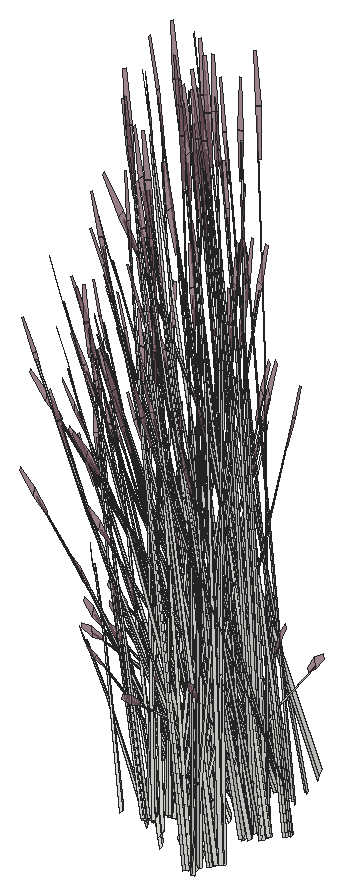
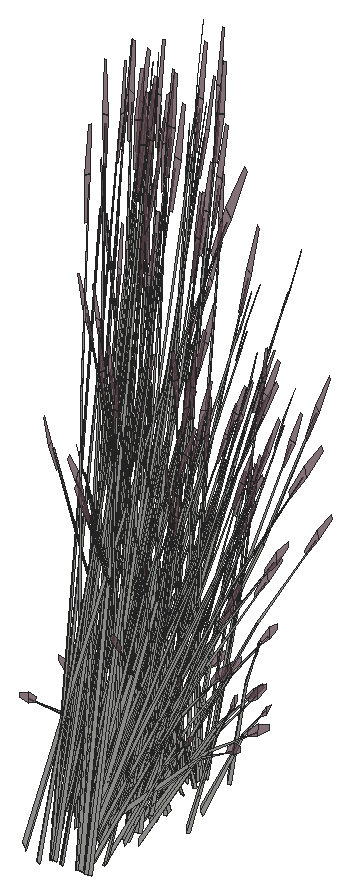
# SketchUp Ruby script. Lengths in inches.
U = 1.inch
M = Sketchup.active_model
def pt(a) = Geom::Point3d.new(a.map { |v| v * U })
def face(e, loops, mat)
  f = e.add_face(loops[0].map { |a| pt(a) })
  loops[1..].each { |l| e.add_face(l.map { |a| pt(a) }).erase! }
  f.material = f.back_material = mat if mat
  f
end
# faces: each face lists its corners as indices into pts; further lists are holes
def faces(e, pts, list, mat = nil) = list.each { |f| face(e, (f[0].is_a?(Array) ? f : [f]).map { |l| l.map { |i| pts[i] } }, mat) }
# xy, xz, yz: faces in a plane at the given z, y or x. An outline is a flat list of corners, or four numbers for a rectangle; further outlines are holes
def ring(l) = l.size == 4 ? [[l[0], l[1]], [l[2], l[1]], [l[2], l[3]], [l[0], l[3]]] : l.each_slice(2).to_a
def flat(e, list, mat, &to3) = list.each { |f| face(e, (f[0].is_a?(Array) ? f : [f]).map { |l| ring(l).map { |u, v| to3.(u, v) } }, mat) }
def xy(e, z, list, mat = nil) = flat(e, list, mat) { |x, y| [x, y, z] }
def xz(e, y, list, mat = nil) = flat(e, list, mat) { |x, z| [x, y, z] }
def yz(e, x, list, mat = nil) = flat(e, list, mat) { |y, z| [x, y, z] }
def lines(e, pts, list) = list.each { |a, b| e.add_line(pt(pts[a]), pt(pts[b])) }
# prism: a flat outline (further loops are holes) pulled along v
def prism(e, loops, v, mat = nil)
  f = face(e, loops, mat); d = Geom::Vector3d.new(v.map { |x| x * U })
  f.pushpull(f.normal.samedirection?(d) ? d.length : -d.length)
end
def box(e, o, s, mat = nil) = prism(e, [[o, [o[0] + s[0], o[1], o[2]], [o[0] + s[0], o[1] + s[1], o[2]], [o[0], o[1] + s[1], o[2]]]], [0, 0, s[2]], mat)
def at(x, y, z, deg = 0) = Geom::Transformation.translation(pt([x, y, z])) * Geom::Transformation.rotation(ORIGIN, Z_AXIS, deg.degrees)
def axes(o, x, y, z) = Geom::Transformation.new([*x, 0, *y, 0, *z, 0, *pt(o).to_a, 1])
def part(name) = M.definitions.add(name)
# library, detail: a bought-in or finely detailed component or shape, given as its bounding box
def library(name, o, s) = part(name).tap { |d| box(d.entities, o, s) }
def detail(e, o, s) = box(e.add_group.entities, o, s)
def put(e, d, t, mat = nil) = e.add_instance(d, t).tap { |i| i.material = mat if mat }
def group(e, t, mat = nil) = e.add_group.tap { |g| g.transformation = t; g.material = mat if mat }.entities
root = M.entities
M.materials.add("LightPink_Translucent").color = [144, 107, 117]
M.materials["LightPink_Translucent"].alpha = 0.75
c1 = part("blade")
p = [[2.15,0.21,22],[0,0.17,0],[0.09,0.45,0],[2.18,0.31,22],[2.29,0.31,22],[0.38,0.45,0],
  [2.48,0.24,33],[2.49,0.24,33],[2.48,0.22,33]]
faces(c1.entities,p,[[0,1,2,3],[4,5,2,3],[6,3,4,7],[8,0,3,6]])
c2 = part("seeds")
p = [[0.3,-0.1,1.38],[-0.01,-0.03,1.59],[-0.01,-0.03,0.03],[0.14,-0.07,-0.07],[0.29,-0.03,3],[0.15,0.01,3.11]]
faces(c2.entities,p,[[0,1,2,3],[1,0,4,5]],"LightPink_Translucent")
c3 = part("blade with seeds")
put(c3.entities,c1,at(0,0,0))
put(c3.entities,c2,axes([2.4,0.25,30.99],[1.5799,-0.05474,1.17369],[-0.12525,1.92788,0.29478],[-0.07173,-0.02425,1.56792]))
put(root,c3,axes([686.68,316.59,393.22],[0.22574,-0.12077,1.42242],[0.19004,0.55807,0.11501],[-0.35439,0.12613,0.60807]))
put(root,c3,axes([686.59,320.47,394.13],[-0.65035,-0.01375,-0.58968],[0.04368,-0.5789,0.07116],[-0.27552,-0.06109,0.83415]))
put(root,c3,axes([683.64,311.58,393.91],[0.08303,0.01531,1.47228],[0.25685,0.50448,-0.13912],[-0.16996,0.13241,0.26054]))
put(root,c3,axes([686.0625,320.61,392.15],[0.12702,0.15896,1.18691],[-0.2927,0.4321,-0.25526],[-0.30054,-0.10328,0.50747]))
put(root,c3,axes([685.97,317.54,392.15],[0.2261,0.04687,1.18691],[0.14573,0.47875,-0.25526],[-0.30712,0.08962,0.50747]))
put(root,c3,axes([686.29,320.09,393.22],[0.24166,0.09837,1.42242],[-0.50011,0.41269,0.11501],[-0.3117,-0.18617,0.60807]))
put(root,c3,axes([687.97,316.01,392.77],[0.18493,-0.0826,1.46963],[0.06377,0.5767,0.11501],[-0.40056,0.07652,0.52526]))
put(root,c3,axes([684.33,313.1875,392.3],[0.27113,-0.25877,0.95334],[0.10699,0.40966,0.70045],[-0.19594,0.07335,0.20998]))
put(root,c3,axes([686.37,320.59,393.89],[-0.47241,0.37822,-0.42412],[-0.41372,-0.39954,-0.32852],[-0.24002,-0.05755,0.81151]))
put(root,c3,axes([685.99,316.39,393.91],[-0.10624,0.07413,1.45204],[0.00904,0.54162,-0.22964],[-0.24352,0.07044,0.11645]))
put(root,c3,axes([687.37,315.08,394.13],[-0.65035,-0.01375,-0.58968],[0.04368,-0.5789,0.07116],[-0.27552,-0.06109,0.83415]))
put(root,c3,axes([685.7,319.53,393.91],[0.04823,0.05698,1.47228],[-0.23252,0.51221,-0.13912],[-0.23548,0.00371,0.26054]))
put(root,c3,axes([686.85,315.22,392.15],[0.12702,0.15896,1.18691],[-0.2927,0.4321,-0.25526],[-0.30054,-0.10328,0.50747]))
put(root,c3,axes([686.33,311.61,393.22],[0.1625,-0.17544,1.42242],[0.41029,0.47354,0.11501],[-0.28141,0.21565,0.60807]))
put(root,c3,axes([685.36,312.07,393.76],[-0.56631,0.0816,-0.29394],[-0.14954,-0.46647,0.37948],[-0.16229,0.12529,0.72609]))
put(root,c3,axes([686.33,316.09,393.76],[-0.54068,-0.15928,-0.29394],[0.1577,-0.46469,0.37948],[-0.21769,0.04261,0.72609]))
put(root,c3,axes([686.24,319.19,393.91],[-0.13998,-0.00403,1.45204],[-0.44565,0.40302,-0.22964],[-0.23779,-0.08235,0.11645]))
put(root,c3,axes([685.05,313.45,391.24],[0.08727,0.05704,1.46364],[0.14797,0.52853,-0.2236],[-0.19341,0.11271,0.24931]))
put(root,c3,axes([686.2,320.23,393.76],[-0.37017,-0.35748,-0.29394],[0.42268,-0.3384,0.37948],[-0.21476,-0.05149,0.72609]))
put(root,c3,axes([684.81,316.94,393.91],[0.08303,0.01531,1.47228],[0.25685,0.50448,-0.13912],[-0.16996,0.13241,0.26054]))
put(root,c3,axes([686.7,316.32,393.89],[-0.17625,0.51936,-0.42412],[-0.60429,-0.17802,-0.32852],[-0.2433,0.04762,0.81151]))
put(root,c3,axes([685.43,311.97,393.93],[-0.16135,-0.52549,0.39842],[0.63294,-0.0912,0.32852],[-0.18654,0.12359,0.82444]))
put(root,c3,axes([687.16,315.2,393.89],[-0.47241,0.37822,-0.42412],[-0.41372,-0.39954,-0.32852],[-0.24002,-0.05755,0.81151]))
put(root,c3,axes([686.39,316.29,391.24],[0.0165,0.08998,1.46364],[-0.33262,0.46992,-0.2236],[-0.23626,-0.02369,0.24931]))
put(root,c3,axes([685.3,311.87,393.93],[-0.44663,-0.24013,0.05337],[0.26003,-0.34195,0.42015],[-0.14319,0.11055,0.64067]))
put(root,c3,axes([686.49,314.14,393.91],[0.04823,0.05698,1.47228],[-0.23252,0.51221,-0.13912],[-0.23548,0.00371,0.26054]))
put(root,c3,axes([686.21,312.04,393.22],[0.12114,-0.19625,1.42242],[0.50818,0.40613,0.11501],[-0.22925,0.25313,0.60807]))
put(root,c3,axes([685.5,318.54,392.3],[0.27113,-0.25877,0.95334],[0.10699,0.40966,0.70045],[-0.19594,0.07335,0.20998]))
put(root,c3,axes([686.14,320.1,394.23],[0.53728,-0.42137,0.44623],[0.46337,0.44748,0.36794],[-0.25207,-0.07773,0.92337]))
put(root,c3,axes([686.45,316.03,393.93],[0.18381,-0.5206,0.39842],[0.60429,0.17802,0.32852],[-0.23764,0.03129,0.82444]))
put(root,c3,axes([686.67,315.88,394.18],[0.32734,0.51701,-0.10093],[-0.58097,0.25407,-0.56021],[-0.24483,0.06821,0.85122]))
put(root,c3,axes([687.4,314.8,394.18],[-0.03484,0.58066,-0.10093],[-0.65957,-0.01587,-0.56021],[-0.25402,-0.04034,0.85122]))
put(root,c3,axes([686.98,314.84,393.76],[-0.37017,-0.35748,-0.29394],[0.42268,-0.3384,0.37948],[-0.21476,-0.05149,0.72609]))
put(root,c3,axes([685.82,312.12,393.89],[0.16713,0.52135,-0.42412],[-0.63294,0.0912,-0.32852],[-0.18138,0.14003,0.81151]))
put(root,c3,axes([686.41,315.89,393.93],[-0.23895,-0.38931,0.05337],[0.43573,-0.19055,0.42015],[-0.19208,0.0376,0.64067]))
put(root,c3,axes([684.83,313.06,393.91],[-0.01617,0.11299,1.45204],[0.45894,0.39307,-0.22964],[-0.12015,0.18588,0.11645]))
put(root,c3,axes([686.52,317.43,393.76],[-0.56631,0.0816,-0.29394],[-0.14954,-0.46647,0.37948],[-0.16229,0.12529,0.72609]))
put(root,c3,axes([686.09,315.7,392.3],[0.41536,-0.04086,0.95334],[-0.26347,0.35999,0.70045],[-0.20525,-0.054,0.20998]))
put(root,c3,axes([686.39,320.09,393.93],[0.03276,-0.43418,0.05337],[0.49468,0.0119,0.42015],[-0.18949,-0.04543,0.64067]))
put(root,c3,axes([686.6,317.32,393.93],[-0.16135,-0.52549,0.39842],[0.63294,-0.0912,0.32852],[-0.18654,0.12359,0.82444]))
put(root,c3,axes([687.91,319.34,394.51],[-0.4342,0.54737,-0.11304],[-0.6288,-0.31535,-0.62743],[-0.21858,-0.15465,0.95337]))
put(root,c3,axes([686.92,314.71,394.23],[0.53728,-0.42137,0.44623],[0.46337,0.44748,0.36794],[-0.25207,-0.07773,0.92337]))
put(root,c3,axes([685.52,311.75,394.18],[0.60181,0.31483,-0.10093],[-0.34671,0.45593,-0.56021],[-0.17003,0.15849,0.85122]))
put(root,c3,axes([686.72,320.42,394.19],[0.37017,0.35748,0.29394],[-0.42268,0.3384,-0.37948],[-0.21476,-0.05149,0.72609]))
put(root,c3,axes([686.47,317.22,393.93],[-0.44663,-0.24013,0.05337],[0.26003,-0.34195,0.42015],[-0.14319,0.11055,0.64067]))
put(root,c3,axes([687.72,319.79,394.13],[-0.55475,-0.27598,-0.58968],[0.39425,-0.48361,0.07116],[-0.20099,-0.16478,0.83415]))
put(root,c3,axes([687.46,319.8,393.89],[-0.64198,0.13573,-0.42412],[-0.1123,-0.514,-0.32852],[-0.17243,-0.1473,0.81151]))
put(root,c3,axes([686.63,319.33,391.24],[-0.06302,0.07522,1.46364],[-0.63686,0.16217,-0.2236],[-0.15385,-0.14752,0.24931]))
put(root,c3,axes([684.53,313.12,394.6875],[0.5741,0.15241,-0.05385],[-0.1766,0.46909,-0.24415],[-0.0939,0.07122,0.8053]))
put(root,c3,axes([686.9,316.03,394.19],[0.54068,0.15928,0.29394],[-0.1577,0.46469,-0.37948],[-0.21769,0.04261,0.72609]))
put(root,c3,axes([685.82,311.79,394.19],[0.56631,-0.0816,0.29394],[0.14954,0.46647,-0.37948],[-0.16229,0.12529,0.72609]))
put(root,c3,axes([686.14,314.01,392.15],[0.2053,-0.09007,1.18691],[0.50689,0.27159,-0.25526],[-0.15087,0.235,0.50747]))
put(root,c3,axes([687.17,314.71,393.93],[0.03276,-0.43418,0.05337],[0.49468,0.0119,0.42015],[-0.18949,-0.04543,0.64067]))
put(root,c3,axes([688.57,317.11,391.71],[-0.67676,-0.09361,-0.51753],[0.14281,-0.57742,-0.13583],[-0.20196,-0.06997,1.14236]))
put(root,c3,axes([687.51,315.03,394.19],[0.37017,0.35748,0.29394],[-0.42268,0.3384,-0.37948],[-0.21476,-0.05149,0.72609]))
put(root,c3,axes([686.35,313.03,393.93],[-0.46327,-0.38957,0.39842],[0.49199,-0.33598,0.32852],[-0.08546,0.18277,0.82444]))
put(root,c3,axes([686.23,319.62,391.77],[-0.18768,0.46622,-0.03231],[-0.57763,-0.14342,-0.14649],[-0.0877,-0.07626,0.48318]))
put(root,c3,axes([687.68,318.2,391.67],[-0.60889,-0.28548,-0.4121],[0.36394,-0.51192,0],[-0.13868,-0.06502,1.30728]))
put(root,c3,axes([686.18,312.99,393.93],[-0.53464,-0.0266,0.05337],[0.01466,-0.40172,0.42015],[-0.05594,0.15388,0.64067]))
put(root,c3,axes([687.74,318.04,393.91],[-0.01214,0.06844,1.47228],[-0.59861,0.24837,-0.13912],[-0.17615,-0.12696,0.26054]))
put(root,c3,axes([686.35,313.15,393.76],[-0.4402,0.30062,-0.29394],[-0.41671,-0.34326,0.37948],[-0.0634,0.1744,0.72609]))
put(root,c3,axes([687.1,319.04,392.15],[-0.0394,0.18678,1.18691],[-0.57594,0.15636,-0.25526],[-0.13463,-0.24142,0.50747]))
put(root,c3,axes([688.05,318.54,391.97],[-0.40676,0.57214,0],[-0.68052,-0.31907,-0.42834],[-0.15499,-0.07267,1.3588]))
put(root,c3,axes([687.29,319.52,393.22],[0.14872,0.18332,1.42242],[-0.6872,0.15433,0.11501],[-0.15531,-0.28779,0.60807]))
put(root,c3,axes([688.6,312.25,391.71],[-0.43821,0.42916,-0.51753],[-0.54436,-0.38915,-0.13583],[-0.1756,0.10706,1.14236]))
put(root,c3,axes([687.53,319.42,393.76],[-0.10048,-0.4599,-0.29394],[0.5744,-0.12144,0.37948],[-0.15428,-0.13179,0.72609]))
put(root,c3,axes([685.92,321.75,391.97],[-0.81352,0,0],[0,-0.63814,-0.42834],[0,-0.14534,1.3588]))
put(root,c3,axes([684.78,314.22,393.91],[0.07381,-0.03447,1.47228],[0.61004,0.22929,-0.13912],[-0.01434,0.19091,0.26054]))
put(root,c3,axes([685.7,318.47,394.6875],[0.5741,0.15241,-0.05385],[-0.1766,0.46909,-0.24415],[-0.0939,0.07122,0.8053]))
put(root,c3,axes([686.99,317.15,394.19],[0.56631,-0.0816,0.29394],[0.14954,0.46647,-0.37948],[-0.16229,0.12529,0.72609]))
put(root,c3,axes([687.02,314.24,391.77],[-0.18768,0.46622,-0.03231],[-0.57763,-0.14342,-0.14649],[-0.0877,-0.07626,0.48318]))
put(root,c3,axes([687.87,319.8,394.19],[0.10048,0.4599,0.29394],[-0.5744,0.12144,-0.37948],[-0.15428,-0.13179,0.72609]))
put(root,c3,axes([686.65,312.83,394.43],[-0.01693,0.52814,-0.65454],[-0.71285,-0.03547,0.07899],[-0.07523,0.22375,0.92591]))
put(root,c3,axes([686.55,321.58,391.93],[-0.60515,0.48003,0.25528],[-0.60552,-0.47498,-0.30288],[-0.02113,-0.13632,1.36855]))
put(root,c3,axes([686.63,314.32,392.3],[-0.01684,-0.3395,0.95334],[0.42072,0.24214,0.70045],[-0.08274,0.16182,0.20998]))
put(root,c3,axes([688.58,311.91,391.83],[-0.70648,0.03525,-0.37133],[-0.06389,-0.58508,0.17871],[-0.12647,0.0593,1.19224]))
put(root,c3,axes([689.05,322.91,392.76],[0.56221,0.23024,1.25546],[-0.55078,0.49601,0.49647],[-0.2467,-0.29398,1.05249]))
put(root,c3,axes([689.34,317.19,392.21],[-0.65687,0.37907,-0.24149],[-0.43681,-0.53562,-0.41502],[-0.16207,-0.0544,1.32557]))
put(root,c3,axes([686.9,318.73,392.3],[0.33937,0.19872,0.95334],[-0.49424,0.11946,0.70045],[-0.10575,-0.15273,0.20998]))
put(root,c3,axes([686.71,316.36,391.97],[-0.81352,0,0],[0,-0.63814,-0.42834],[0,-0.14534,1.3588]))
put(root,c3,axes([687.85,317.99,391.68],[-0.15283,-0.49751,-0.25712],[0.60696,-0.14127,0.25712],[-0.12236,-0.05737,1.15348]))
put(root,c3,axes([686.41,313.57,392.79],[0.01429,-0.29475,1.28107],[0.64291,0.15569,0.17703],[-0.0557,0.31414,0.60492]))
put(root,c3,axes([687.61,319.26,394.23],[0.72473,-0.14676,0.44623],[0.12578,0.57568,0.36794],[-0.17045,-0.16967,0.92337]))
put(root,c3,axes([687.77,319.38,393.93],[0.29569,-0.36271,0.05337],[0.42107,0.21117,0.42015],[-0.13613,-0.11629,0.64067]))
put(root,c3,axes([689.33,313.42,391.67],[-0.60889,0.28548,-0.4121],[-0.36394,-0.51192,0],[-0.13868,0.06502,1.30728]))
put(root,c3,axes([689.37,313.26,391.82],[-0.40169,-0.57414,-0.04268],[0.68052,-0.31907,0.42834],[-0.16769,0.05466,1.35813]))
put(root,c3,axes([687.34,316.2,391.93],[-0.60515,0.48003,0.25528],[-0.60552,-0.47498,-0.30288],[-0.02113,-0.13632,1.36855]))
put(root,c3,axes([688.19,322.58,392.02],[0.17244,-0.67657,-0.19446],[0.81759,0.11793,0.42555],[-0.14286,-0.09343,1.29846]))
put(root,c3,axes([686.79,313.01,394.15],[0.46573,0.38364,-0.47077],[-0.49199,0.33598,-0.36465],[-0.07086,0.19492,0.90078]))
put(root,c3,axes([689.18,313.19,391.68],[-0.60696,-0.14127,-0.25712],[0.15283,-0.49751,0.25712],[-0.12236,0.05737,1.15348]))
put(root,c3,axes([686.58,312.72,394.19],[0.4402,-0.30062,0.29394],[0.41671,0.34326,-0.37948],[-0.0634,0.1744,0.72609]))
put(root,c3,axes([690.07,317.36,392.05],[-0.63528,-0.45956,-0.20909],[0.53456,-0.51604,0.45758],[-0.17107,0.05376,1.39619]))
put(root,c3,axes([688.92,316.92,391.83],[-0.39083,-0.47924,-0.37133],[0.59199,-0.33747,0.17871],[-0.12647,-0.0593,1.19224]))
put(root,c3,axes([688.42,318.3,393.91],[-0.09951,-0.08005,1.45204],[-0.66407,0.05075,-0.22964],[-0.10598,-0.19148,0.11645]))
put(root,c3,axes([689.53,311.06,392.36],[-0.01777,-0.53759,1.17256],[0.80434,0.13935,0.49647],[-0.19024,0.29416,1.1068]))
put(root,c3,axes([686.11,321.32,391.67],[0,-0.57097,-0.4121],[0.72788,0,0],[0,-0.13004,1.30728]))
put(root,c3,axes([686.3,312.8,394.48],[0.71502,0.02829,-0.11203],[-0.01954,0.53563,-0.62183],[-0.04967,0.20629,0.94486]))
put(root,c3,axes([689.75,317.27,391.83],[-0.70648,0.03525,-0.37133],[-0.06389,-0.58508,0.17871],[-0.12647,0.0593,1.19224]))
put(root,c3,axes([686.28,313.58,392.34],[0.59102,-0.10111,0.05401],[0.13587,0.40735,-0.71633],[-0.03747,0.2062,0.64209]))
put(root,c3,axes([689.08,311.75,392.21],[0.07581,0.65151,-0.24149],[-0.7896,0.03939,-0.41502],[-0.13904,0.08678,1.32557]))
put(root,c3,axes([688.01,321.98,392.21],[-0.73268,-0.27244,-0.24149],[0.35279,-0.57501,-0.41502],[-0.02303,-0.14118,1.32557]))
put(root,c3,axes([687.32,312.46,393.22],[-0.01592,-0.21915,1.42242],[0.69015,0.14538,0.11501],[-0.04269,0.3123,0.60807]))
put(root,c3,axes([688.4,318.24,392.06],[0.60889,0.28548,0.4121],[-0.36394,0.51192,0],[-0.13868,-0.06502,1.30728]))
put(root,c3,axes([688.98,317.2,392.02],[0.17244,-0.67657,-0.19446],[0.81759,0.11793,0.42555],[-0.14286,-0.09343,1.29846]))
put(root,c3,axes([687.68,321.4,391.74],[-0.26718,-0.5855,-0.57963],[0.76964,-0.21087,-0.15213],[-0.02953,-0.19827,1.27944]))
put(root,c3,axes([689.43,319.54,394.18],[-0.63664,0.26583,-0.10093],[-0.31286,-0.47181,-0.56021],[-0.084,-0.19882,0.85122]))
put(root,c3,axes([688.88,319.5625,393.89],[-0.63954,-0.14313,-0.42412],[0.21921,-0.49074,-0.32852],[-0.05864,-0.19758,0.81151]))
put(root,c3,axes([689.27,317.36,392.17],[-0.12551,0.50956,0.12018],[-0.6132,-0.08845,-0.34318],[-0.1116,-0.05232,1.05198]))
put(root,c3,axes([687.2,316.46,392.06],[0,0.57097,0.4121],[-0.72788,0,0],[0,-0.13004,1.30728]))
put(root,c3,axes([690.54,318.625,391.82],[-0.40169,-0.57414,-0.04268],[0.68052,-0.31907,0.42834],[-0.16769,0.05466,1.35813]))
put(root,c3,axes([686.42,321.33,391.68],[0.45414,-0.35624,-0.25712],[0.45414,0.35624,0.25712],[0,-0.11474,1.15348]))
put(root,c3,axes([688.47,319.03,391.77],[-0.44958,0.32756,-0.03231],[-0.41194,-0.35875,-0.14649],[-0.029,-0.10165,0.48318]))
put(root,c3,axes([690.35,318.55,391.68],[-0.60696,-0.14127,-0.25712],[0.15283,-0.49751,0.25712],[-0.12236,0.05737,1.15348]))
put(root,c3,axes([688.79,316.59,392.21],[-0.73268,-0.27244,-0.24149],[0.35279,-0.57501,-0.41502],[-0.02303,-0.14118,1.32557]))
put(root,c3,axes([689.12,319.66,394.13],[-0.31051,-0.46426,-0.58968],[0.63919,-0.25873,0.07116],[-0.07261,-0.22432,0.83415]))
put(root,c3,axes([689.88,313.33,391.97],[0.40676,0.57214,0],[-0.68052,0.31907,-0.42834],[-0.15499,0.07267,1.3588]))
put(root,c3,axes([687.81,313.58,394.2],[-0.64106,-0.14927,0.44225],[0.21921,-0.49074,0.36465],[0.03852,0.19299,0.91512]))
put(root,c3,axes([690.25,317.11,392.21],[0.07581,0.65151,-0.24149],[-0.7896,0.03939,-0.41502],[-0.13904,0.08678,1.32557]))
put(root,c3,axes([687.64,313.61,393.93],[-0.47939,0.19405,0.05337],[-0.23464,-0.35385,0.42015],[0.0463,0.15598,0.64067]))
put(root,c3,axes([689.22,311.875,392.17],[0.48065,0.34305,0.12018],[-0.40092,0.38703,-0.34318],[-0.1116,0.05232,1.05198]))
put(root,c3,axes([689.24,319.72,394.19],[-0.19614,0.43908,0.29394],[-0.57222,-0.12807,-0.37948],[-0.05247,-0.17678,0.72609]))
put(root,c3,axes([687.2,315.94,391.68],[0.45414,-0.35624,-0.25712],[0.45414,0.35624,0.25712],[0,-0.11474,1.15348]))
put(root,c3,axes([689.07,316.87,391.96],[0.82229,0.1203,0.37976],[-0.16734,0.67942,0.14902],[-0.12017,-0.06561,1.31851]))
put(root,c3,axes([689.38,312.97,391.93],[0.81449,0.18558,0.25528],[-0.20377,0.66335,-0.30288],[-0.13481,0.08302,1.36855]))
put(root,c3,axes([689.74,312.93,392.06],[0.60889,-0.28548,0.4121],[0.36394,0.51192,0],[-0.13868,0.06502,1.30728]))
put(root,c3,axes([688.86,316.75,392.26],[-0.31565,0.51449,0.37133],[-0.65588,-0.24761,-0.17871],[0,-0.1186,1.19224]))
put(root,c3,axes([687.74,313.5,391.24],[0.10529,-0.03107,1.46364],[0.63335,0.17101,-0.2236],[0.01852,0.19274,0.24931]))
put(root,c3,axes([687.88,313.68,393.76],[-0.19614,0.43908,-0.29394],[-0.57222,-0.12807,0.37948],[0.05247,0.17678,0.72609]))
put(root,c3,axes([688.58,318.625,391.24],[-0.10912,0.02057,1.46364],[-0.60346,-0.23156,-0.2236],[0.01013,-0.19315,0.24931]))
put(root,c3,axes([688.63,317.96,392.05],[0.6991,-0.15154,0.14643],[0.17263,0.56398,0.29122],[-0.06235,-0.08217,1.33138]))
put(root,c3,axes([689.18,319.26,393.76],[0.19614,-0.43908,-0.29394],[0.57222,0.12807,0.37948],[-0.05247,-0.17678,0.72609]))
put(root,c3,axes([689.53,318.05,391.82],[-0.65588,-0.25634,0],[0.31565,-0.53263,0],[0,0,1.35047]))
put(root,c3,axes([688.09,321.55,391.83],[0.31565,-0.51449,-0.37133],[0.65588,0.24761,0.17871],[0,-0.1186,1.19224]))
put(root,c3,axes([689.37,311.49,391.83],[-0.31565,0.51449,-0.37133],[-0.65588,-0.24761,0.17871],[0,0.1186,1.19224]))
put(root,c3,axes([687.47,314.46,393.91],[0.08247,0.09194,1.45204],[0.66552,0.03612,-0.22964],[0.06692,0.20277,0.11645]))
put(root,c3,axes([690.71,317.99,392.05],[0.18794,-0.56744,0.14643],[0.68774,0.16058,0.29122],[-0.1188,0.00276,1.33138]))
